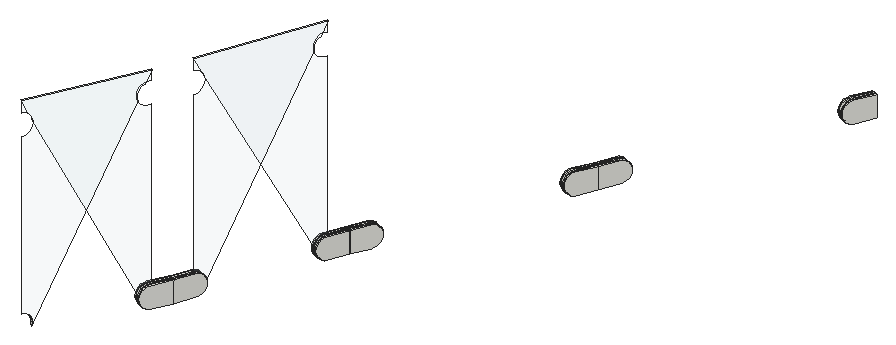
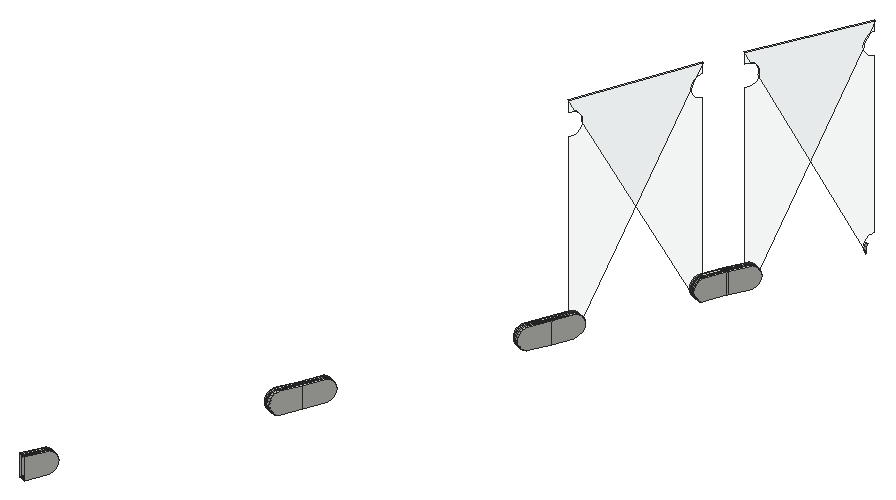
# SketchUp Ruby script. Lengths in inches.
U = 1.inch
M = Sketchup.active_model
def pt(a) = Geom::Point3d.new(a.map { |v| v * U })
def face(e, loops, mat)
  f = e.add_face(loops[0].map { |a| pt(a) })
  loops[1..].each { |l| e.add_face(l.map { |a| pt(a) }).erase! }
  f.material = f.back_material = mat if mat
  f
end
# faces: each face lists its corners as indices into pts; further lists are holes
def faces(e, pts, list, mat = nil) = list.each { |f| face(e, (f[0].is_a?(Array) ? f : [f]).map { |l| l.map { |i| pts[i] } }, mat) }
# xy, xz, yz: faces in a plane at the given z, y or x. An outline is a flat list of corners, or four numbers for a rectangle; further outlines are holes
def ring(l) = l.size == 4 ? [[l[0], l[1]], [l[2], l[1]], [l[2], l[3]], [l[0], l[3]]] : l.each_slice(2).to_a
def flat(e, list, mat, &to3) = list.each { |f| face(e, (f[0].is_a?(Array) ? f : [f]).map { |l| ring(l).map { |u, v| to3.(u, v) } }, mat) }
def xy(e, z, list, mat = nil) = flat(e, list, mat) { |x, y| [x, y, z] }
def xz(e, y, list, mat = nil) = flat(e, list, mat) { |x, z| [x, y, z] }
def yz(e, x, list, mat = nil) = flat(e, list, mat) { |y, z| [x, y, z] }
def lines(e, pts, list) = list.each { |a, b| e.add_line(pt(pts[a]), pt(pts[b])) }
# prism: a flat outline (further loops are holes) pulled along v
def prism(e, loops, v, mat = nil)
  f = face(e, loops, mat); d = Geom::Vector3d.new(v.map { |x| x * U })
  f.pushpull(f.normal.samedirection?(d) ? d.length : -d.length)
end
def box(e, o, s, mat = nil) = prism(e, [[o, [o[0] + s[0], o[1], o[2]], [o[0] + s[0], o[1] + s[1], o[2]], [o[0], o[1] + s[1], o[2]]]], [0, 0, s[2]], mat)
def at(x, y, z, deg = 0) = Geom::Transformation.translation(pt([x, y, z])) * Geom::Transformation.rotation(ORIGIN, Z_AXIS, deg.degrees)
def axes(o, x, y, z) = Geom::Transformation.new([*x, 0, *y, 0, *z, 0, *pt(o).to_a, 1])
def part(name) = M.definitions.add(name)
# library, detail: a bought-in or finely detailed component or shape, given as its bounding box
def library(name, o, s) = part(name).tap { |d| box(d.entities, o, s) }
def detail(e, o, s) = box(e.add_group.entities, o, s)
def put(e, d, t, mat = nil) = e.add_instance(d, t).tap { |i| i.material = mat if mat }
def group(e, t, mat = nil) = e.add_group.tap { |g| g.transformation = t; g.material = mat if mat }.entities
root = M.entities
M.materials.add("Glass_Safety_01").color = [204, 235, 244]
M.materials["Glass_Safety_01"].alpha = 0.1
xy(root,333,[[882.822,624.661,882.573,624.779,882.681,625.009,883.414,626.559,883.663,626.441],[882.395,624.863,882.145,624.981,882.977,626.738,883.233,626.637,882.503,625.093],[883.672,626.464,883.416,626.565,884.14,628.396,884.396,628.294],[883.233,626.637,882.977,626.738,882.981,626.75,882.986,626.761,883.236,626.643],[883.236,626.643,882.986,626.761,883.7,628.569,883.957,628.468],
  [888.84,639.54,888.584,639.641,888.672,639.866,889.306,641.468,889.558,641.358],[888.4,639.713,888.144,639.814,888.868,641.645,889.124,641.544,888.489,639.938],[889.558,641.358,889.306,641.468,889.307,641.472,889.563,641.37,889.561,641.364],[889.563,641.37,889.307,641.472,890.092,643.273,890.344,643.163],[889.125,641.547,888.873,641.657,889.659,643.462,889.911,643.352],
  [897.674,659.993,897.421,660.103,897.491,660.262,898.207,661.907,898.46,661.797],[897.241,660.181,896.988,660.291,897.774,662.096,898.027,661.986,897.31,660.341],[898.46,661.797,898.207,661.907,898.994,663.712,899.246,663.602],[898.027,661.986,897.774,662.096,898.56,663.901,898.813,663.791],[907.619,682.827,907.367,682.937,907.429,683.08,908.153,684.742,908.405,684.632],
  [907.186,683.016,906.933,683.126,907.719,684.93,907.972,684.82,907.248,683.158]])
xy(root,333.078,[[882.741,625.135,882.563,625.219,883.233,626.637,883.325,626.601,883.414,626.559],[883.416,626.565,883.325,626.601,883.236,626.643,883.812,628.102,883.995,628.029],[883.325,626.601,883.233,626.637,883.234,626.64,883.236,626.643],[888.728,640.007,888.545,640.079,889.124,641.544,889.215,641.508,889.306,641.468],[889.306,641.468,889.215,641.508,889.307,641.472,889.306,641.47],
  [889.307,641.472,889.215,641.508,889.125,641.547,889.754,642.991,889.935,642.912],[897.579,660.464,897.398,660.542,898.027,661.986,898.207,661.907],[898.207,661.907,898.027,661.986,898.656,663.43,898.836,663.351],[907.524,683.298,907.343,683.377,907.972,684.82,908.153,684.742]],"Glass_Safety_01")
xy(root,335.047,[[882.741,625.135,883.414,626.559,883.325,626.601,883.233,626.637,882.563,625.219],[883.416,626.565,883.995,628.029,883.812,628.102,883.236,626.643,883.325,626.601],[883.325,626.601,883.236,626.643,883.234,626.64,883.233,626.637],[888.728,640.007,889.306,641.468,889.215,641.508,889.124,641.544,888.545,640.079],[889.306,641.468,889.306,641.47,889.307,641.472,889.215,641.508],
  [889.307,641.472,889.935,642.912,889.754,642.991,889.125,641.547,889.215,641.508],[897.579,660.464,898.207,661.907,898.027,661.986,897.398,660.542],[898.207,661.907,898.836,663.351,898.656,663.43,898.027,661.986]],"Glass_Safety_01")
xy(root,335.126,[[882.822,624.661,883.663,626.441,883.414,626.559,882.681,625.009,882.573,624.779],[882.395,624.863,882.503,625.093,883.233,626.637,882.977,626.738,882.145,624.981],[883.672,626.464,884.396,628.294,884.14,628.396,883.416,626.565],[883.233,626.637,883.236,626.643,882.986,626.761,882.981,626.75,882.977,626.738],[883.236,626.643,883.957,628.468,883.7,628.569,882.986,626.761],
  [888.84,639.54,889.558,641.358,889.306,641.468,888.672,639.866,888.584,639.641],[888.4,639.713,888.489,639.938,889.124,641.544,888.868,641.645,888.144,639.814],[889.558,641.358,889.561,641.364,889.563,641.37,889.307,641.472,889.306,641.468],[889.563,641.37,890.344,643.163,890.092,643.273,889.307,641.472],[889.125,641.547,889.911,643.352,889.659,643.462,888.873,641.657],
  [897.674,659.993,898.46,661.797,898.207,661.907,897.491,660.262,897.421,660.103],[897.241,660.181,897.31,660.341,898.027,661.986,897.774,662.096,896.988,660.291],[898.46,661.797,899.246,663.602,898.994,663.712,898.207,661.907],[898.027,661.986,898.813,663.791,898.56,663.901,897.774,662.096],[907.619,682.827,908.405,684.632,908.153,684.742,907.429,683.08,907.367,682.937],
  [907.186,683.016,907.248,683.158,907.972,684.82,907.719,684.93,906.933,683.126]])
p = [[883.663,626.441,335.126],[882.822,624.661,335.126],[882.704,624.413,335.089],[882.595,624.181,334.983],[882.501,623.982,334.814],[882.428,623.829,334.594],
  [882.383,623.733,334.338],[882.367,623.7,334.0625],[882.383,623.733,333.787],[882.428,623.829,333.531],[882.501,623.982,333.311],[882.595,624.181,333.142],
  [882.704,624.413,333.036],[882.822,624.661,333],[883.663,626.441,333],[882.573,624.779,335.126],[882.681,625.009,335.126],[882.681,625.009,333],
  [882.573,624.779,333],[882.455,624.53,333.036],[882.345,624.299,333.142],[882.251,624.1,333.311],[882.179,623.947,333.531],[882.134,623.851,333.787],
  [882.118,623.818,334.0625],[882.134,623.851,334.338],[882.179,623.947,334.594],[882.251,624.1,334.814],[882.345,624.299,334.983],[882.455,624.53,335.089],
  [882.395,624.863,333],[882.503,625.093,333],[883.233,626.637,333],[883.233,626.637,333.078],[883.233,626.637,335.047],[883.233,626.637,335.126],
  [882.503,625.093,335.126],[882.395,624.863,335.126],[882.277,624.615,335.089],[882.167,624.383,334.983],[882.073,624.184,334.814],[882.001,624.031,334.594],
  [881.962,623.948,334.371],[881.956,623.935,334.338],[881.94,623.902,334.0625],[881.956,623.935,333.787],[882.001,624.031,333.531],[882.073,624.184,333.311],
  [882.167,624.383,333.142],[882.248,624.553,333.064],[882.277,624.615,333.036],[882.145,624.981,335.126],[882.977,626.738,335.126],[882.977,626.738,333],
  [882.145,624.981,333],[882.028,624.732,333.036],[881.918,624.501,333.142],[881.824,624.301,333.311],[881.752,624.149,333.531],[881.707,624.053,333.787],
  [881.691,624.02,334.0625],[881.707,624.053,334.338],[881.752,624.149,334.594],[881.824,624.301,334.814],[881.918,624.501,334.983],[882.028,624.732,335.089],
  [883.414,626.559,333],[883.414,626.559,335.126],[883.414,626.559,335.047],[882.741,625.135,335.047],[882.741,625.135,333.078],[883.414,626.559,333.078],
  [883.416,626.565,333.078],[883.416,626.565,333],[883.672,626.464,333],[883.672,626.464,335.126],[883.416,626.565,335.126],[883.416,626.565,335.047],
  [884.396,628.294,335.126],[884.396,628.294,333],[884.497,628.55,333.036],[884.591,628.789,333.142],[884.672,628.993,333.311],[884.734,629.15,333.531],
  [884.773,629.249,333.787],[884.787,629.283,334.0625],[884.773,629.249,334.338],[884.734,629.15,334.594],[884.672,628.993,334.814],[884.591,628.789,334.983],
  [884.497,628.55,335.089],[883.236,626.643,333.078],[883.236,626.643,333],[882.986,626.761,333],[882.986,626.761,335.126],[883.236,626.643,335.126],
  [883.236,626.643,335.047],[883.957,628.468,333],[884.058,628.724,333.036],[884.152,628.962,333.142],[884.233,629.167,333.311],[884.295,629.324,333.531],
  [884.334,629.423,333.787],[884.347,629.456,334.0625],[884.334,629.423,334.338],[884.295,629.324,334.594],[884.233,629.167,334.814],[884.152,628.962,334.983],
  [884.058,628.724,335.089],[883.957,628.468,335.126],[884.14,628.396,335.126],[884.14,628.396,333],[883.995,628.029,333.078],[883.995,628.029,335.047],
  [882.981,626.75,333],[882.981,626.75,335.126],[883.7,628.569,335.126],[883.801,628.825,335.089],[883.896,629.063,334.983],[883.977,629.268,334.814],
  [884.039,629.425,334.594],[884.078,629.524,334.338],[884.091,629.558,334.0625],[884.078,629.524,333.787],[884.039,629.425,333.531],[883.977,629.268,333.311],
  [883.896,629.063,333.142],[883.801,628.825,333.036],[883.7,628.569,333],[884.241,628.651,333.036],[884.512,629.338,333.756],[884.44,629.157,333.398],
  [884.416,629.095,333.311],[884.335,628.89,333.142],[884.241,628.651,335.089],[884.335,628.89,334.983],[884.416,629.095,334.814],[884.478,629.252,334.594],
  [884.517,629.35,334.338],[884.53,629.384,334.0625],[884.517,629.35,333.787],[888.84,639.54,333],[889.558,641.358,333],[889.558,641.358,335.126],
  [888.84,639.54,335.126],[888.739,639.284,335.089],[888.644,639.045,334.983],[888.564,638.84,334.814],[888.501,638.683,334.594],[888.462,638.585,334.338],
  [888.449,638.551,334.0625],[888.462,638.585,333.787],[888.501,638.683,333.531],[888.564,638.84,333.311],[888.644,639.045,333.142],[888.739,639.284,333.036],
  [888.489,639.938,333],[888.489,639.938,335.126],[888.4,639.713,335.126],[888.299,639.457,335.089],[888.205,639.219,334.983],[888.124,639.014,334.814],
  [888.062,638.857,334.594],[888.023,638.758,334.338],[888.019,638.747,334.245],[888.25,639.332,333.091],[888.299,639.457,333.036],[888.4,639.713,333],
  [888.672,639.866,333],[888.672,639.866,335.126],[888.584,639.641,335.126],[888.482,639.385,335.089],[888.388,639.147,334.983],[888.307,638.942,334.814],
  [888.245,638.785,334.594],[888.206,638.686,334.338],[888.193,638.652,334.0625],[888.206,638.686,333.787],[888.245,638.785,333.531],[888.307,638.942,333.311],
  [888.388,639.147,333.142],[888.482,639.385,333.036],[888.584,639.641,333],[889.306,641.468,335.126],[889.306,641.468,335.047],[889.306,641.468,333.078],
  [889.306,641.468,333],[888.144,639.814,335.126],[888.868,641.645,335.126],[888.868,641.645,333],[888.144,639.814,333],[888.043,639.559,333.036],
  [887.949,639.32,333.142],[887.868,639.115,333.311],[887.806,638.958,333.531],[887.767,638.86,333.787],[887.753,638.826,334.0625],[887.767,638.86,334.338],
  [887.806,638.958,334.594],[887.868,639.115,334.814],[887.949,639.32,334.983],[888.043,639.559,335.089],[888.205,639.219,333.142],[889.124,641.544,335.126],
  [889.124,641.544,333],[889.124,641.544,333.078],[888.545,640.079,333.078],[888.545,640.079,335.047],[889.124,641.544,335.047],[889.307,641.472,333],
  [889.307,641.472,333.078],[889.307,641.472,335.047],[889.307,641.472,335.126],[889.563,641.37,335.126],[889.563,641.37,333],[889.561,641.364,335.126],
  [889.561,641.364,333],[890.344,643.163,333],[890.454,643.415,333.036],[890.557,643.65,333.142],[890.645,643.852,333.311],[890.712,644.007,333.531],
  [890.754,644.105,333.787],[890.769,644.138,334.0625],[890.754,644.105,334.338],[890.712,644.007,334.594],[890.645,643.852,334.814],[890.557,643.65,334.983],
  [890.454,643.415,335.089],[890.344,643.163,335.126],[889.125,641.547,333],[889.125,641.547,333.078],[889.125,641.547,335.047],[889.125,641.547,335.126],
  [888.873,641.657,335.126],[888.873,641.657,333],[889.911,643.352,333],[889.911,643.352,335.126],[889.754,642.991,335.047],[889.754,642.991,333.078],
  [890.092,643.273,335.126],[890.202,643.525,335.089],[890.304,643.76,334.983],[890.392,643.962,334.814],[890.459,644.117,334.594],[890.502,644.215,334.338],
  [890.516,644.248,334.0625],[890.502,644.215,333.787],[890.459,644.117,333.531],[890.392,643.962,333.311],[890.304,643.76,333.142],[890.202,643.525,333.036],
  [890.092,643.273,333],[889.659,643.462,335.126],[889.768,643.714,335.089],[889.871,643.949,334.983],[889.959,644.151,334.814],[890.026,644.306,334.594],
  [890.069,644.403,334.338],[890.083,644.436,334.0625],[890.069,644.403,333.787],[890.026,644.306,333.531],[889.959,644.151,333.311],[889.871,643.949,333.142],
  [889.768,643.714,333.036],[889.659,643.462,333],[890.021,643.604,333.036],[890.021,643.604,335.089],[890.123,643.839,334.983],[890.211,644.041,334.814],
  [890.279,644.196,334.594],[890.321,644.293,334.338],[890.336,644.326,334.0625],[890.321,644.293,333.787],[890.279,644.196,333.531],[890.211,644.041,333.311],
  [890.123,643.839,333.142],[898.46,661.797,335.126],[897.674,659.993,335.126],[897.564,659.74,335.089],[897.462,659.505,334.983],[897.374,659.303,334.814],
  [897.307,659.149,334.594],[897.264,659.051,334.338],[897.25,659.018,334.0625],[897.264,659.051,333.787],[897.307,659.149,333.531],[897.374,659.303,333.311],
  [897.462,659.505,333.142],[897.564,659.74,333.036],[897.674,659.993,333],[898.46,661.797,333],[897.421,660.103,335.126],[897.491,660.262,335.126],
  [897.491,660.262,333],[897.421,660.103,333],[897.312,659.85,333.036],[897.209,659.615,333.142],[897.121,659.414,333.311],[897.054,659.259,333.531],
  [897.011,659.161,333.787],[896.997,659.128,334.0625],[897.011,659.161,334.338],[897.054,659.259,334.594],[897.121,659.414,334.814],[897.209,659.615,334.983],
  [897.312,659.85,335.089],[897.241,660.181,333],[897.31,660.341,333],[897.31,660.341,335.126],[897.241,660.181,335.126],[897.131,659.929,335.089],
  [897.029,659.694,334.983],[896.941,659.492,334.814],[896.873,659.337,334.594],[896.831,659.24,334.338],[896.817,659.207,334.0625],[896.831,659.24,333.787],
  [896.873,659.337,333.531],[896.941,659.492,333.311],[897.029,659.694,333.142],[897.131,659.929,333.036],[896.988,660.291,335.126],[897.774,662.096,335.126],
  [897.774,662.096,333],[896.988,660.291,333],[896.878,660.039,333.036],[896.776,659.804,333.142],[896.688,659.602,333.311],[896.621,659.447,333.531],
  [896.578,659.35,333.787],[896.564,659.317,334.0625],[896.578,659.35,334.338],[896.621,659.447,334.594],[896.688,659.602,334.814],[896.776,659.804,334.983],
  [896.878,660.039,335.089],[898.027,661.986,335.126],[898.027,661.986,333],[898.027,661.986,333.078],[897.398,660.542,333.078],[897.398,660.542,335.047],
  [898.027,661.986,335.047],[898.207,661.907,333],[898.207,661.907,335.126],[898.207,661.907,335.047],[897.579,660.464,335.047],[897.579,660.464,333.078],
  [898.207,661.907,333.078],[899.246,663.602,335.126],[899.246,663.602,333],[899.356,663.854,333.036],[899.458,664.089,333.142],[899.546,664.291,333.311],
  [899.614,664.446,333.531],[899.656,664.543,333.787],[899.671,664.577,334.0625],[899.656,664.543,334.338],[899.614,664.446,334.594],[899.546,664.291,334.814],
  [899.458,664.089,334.983],[899.356,663.854,335.089],[898.994,663.712,335.126],[898.994,663.712,333],[898.836,663.351,333.078],[898.836,663.351,335.047],
  [898.813,663.791,333],[898.813,663.791,335.126],[898.656,663.43,335.047],[898.656,663.43,333.078],[898.56,663.901,335.126],[898.67,664.153,335.089],
  [898.773,664.388,334.983],[898.86,664.59,334.814],[898.928,664.745,334.594],[898.97,664.842,334.338],[898.985,664.875,334.0625],[898.97,664.842,333.787],
  [898.928,664.745,333.531],[898.86,664.59,333.311],[898.773,664.388,333.142],[898.67,664.153,333.036],[898.56,663.901,333],[899.103,663.964,333.036],
  [899.206,664.199,333.142],[899.294,664.401,333.311],[899.361,664.556,333.531],[899.403,664.654,333.787],[899.418,664.687,334.0625],[899.403,664.654,334.338],
  [899.361,664.556,334.594],[899.294,664.401,334.814],[899.206,664.199,334.983],[899.103,663.964,335.089],[898.923,664.043,333.036],[898.923,664.043,335.089],
  [899.025,664.278,334.983],[899.113,664.48,334.814],[899.181,664.635,334.594],[899.223,664.732,334.338],[899.237,664.765,334.0625],[899.223,664.732,333.787],
  [899.181,664.635,333.531],[899.113,664.48,333.311],[899.025,664.278,333.142],[908.405,684.632,335.126],[907.619,682.827,335.126],[907.509,682.575,335.089],
  [907.407,682.34,334.983],[907.319,682.138,334.814],[907.252,681.983,334.594],[907.209,681.886,334.338],[907.195,681.852,334.0625],[907.209,681.886,333.787],
  [907.252,681.983,333.531],[907.319,682.138,333.311],[907.407,682.34,333.142],[907.509,682.575,333.036],[907.619,682.827,333],[908.405,684.632,333],
  [907.186,683.016,333],[907.248,683.158,333],[907.248,683.158,335.126],[907.186,683.016,335.126],[907.076,682.763,335.089],[906.974,682.528,334.983],
  [906.886,682.326,334.814],[906.818,682.172,334.594],[906.776,682.074,334.338],[906.762,682.041,334.0625],[906.776,682.074,333.787],[906.818,682.172,333.531],
  [906.886,682.326,333.311],[906.974,682.528,333.142],[907.076,682.763,333.036],[907.367,682.937,335.126],[907.429,683.08,335.126],[907.429,683.08,333],
  [907.367,682.937,333],[907.257,682.685,333.036],[907.154,682.45,333.142],[907.066,682.248,333.311],[906.999,682.093,333.531],[906.957,681.996,333.787],
  [906.942,681.962,334.0625],[906.957,681.996,334.338],[906.999,682.093,334.594],[907.066,682.248,334.814],[907.154,682.45,334.983],[907.257,682.685,335.089],
  [906.933,683.126,335.126],[907.719,684.93,335.126],[907.719,684.93,333],[906.933,683.126,333],[906.824,682.873,333.036],[906.721,682.638,333.142],
  [906.633,682.437,333.311],[906.566,682.282,333.531],[906.523,682.184,333.787],[906.509,682.151,334.0625],[906.523,682.184,334.338],[906.566,682.282,334.594],
  [906.633,682.437,334.814],[906.721,682.638,334.983],[906.824,682.873,335.089],[908.153,684.742,333],[908.153,684.742,335.126],[908.153,684.742,335.047],
  [907.524,683.298,335.047],[907.524,683.298,333.078],[908.153,684.742,333.078],[907.972,684.82,335.126],[907.972,684.82,333],[907.972,684.82,333.078],
  [907.343,683.377,333.078],[907.343,683.377,335.047],[907.972,684.82,335.047],[882.563,625.219,335.047],[882.563,625.219,333.078],[883.325,626.601,333.078],
  [883.325,626.601,335.047],[883.234,626.64,335.047],[883.234,626.64,333.078],[883.812,628.102,333.078],[883.812,628.102,335.047],[888.01,638.725,334.0625],
  [888.023,638.758,333.787],[888.062,638.857,333.531],[888.124,639.014,333.311],[888.728,640.007,333.078],[888.728,640.007,335.047],[889.215,641.508,335.047],
  [889.215,641.508,333.078],[889.306,641.47,333.078],[889.306,641.47,335.047],[889.935,642.912,335.047],[889.935,642.912,333.078],[884.478,629.252,333.531],
  [878.01,615.586,334.0625],[877.995,615.553,333.787],[877.745,615.671,333.787],[877.761,615.704,334.0625],[884.14,628.396,351.283],[888.202,638.675,352.163],
  [888.193,638.652,352.346],[888.206,638.686,352.621],[888.245,638.785,352.877],[888.307,638.942,353.098],[888.388,639.147,353.267],[888.433,639.26,353.317],
  [888.672,639.866,354.511],[884.14,628.396,354.511],[884.14,628.396,353.409],[884.241,628.651,353.373],[884.335,628.89,353.267],[884.416,629.095,353.098],
  [884.478,629.252,352.877],[884.517,629.35,352.621],[884.53,629.384,352.346],[884.517,629.35,352.071],[884.478,629.252,351.814],[884.416,629.095,351.594],
  [884.335,628.89,351.425],[884.241,628.651,351.319],[878.181,615.487,333.943],[882.14,623.863,352.037],[882.134,623.851,352.071],[882.118,623.818,352.346],
  [882.134,623.851,352.621],[882.179,623.947,352.877],[882.251,624.1,353.098],[882.345,624.299,353.267],[882.426,624.469,353.344],[882.681,625.009,354.511],
  [877.734,614.541,354.511],[877.734,614.541,353.409],[877.851,614.789,353.373],[877.961,615.021,353.267],[878.055,615.22,353.098],[878.127,615.373,352.877],
  [878.173,615.469,352.621],[878.188,615.502,352.346],[878.173,615.469,352.071],[878.127,615.373,351.814],[878.055,615.22,351.594],[877.961,615.021,351.425],
  [877.851,614.789,351.319],[877.734,614.541,351.283],[877.734,614.541,335.126],[877.851,614.789,335.089],[877.961,615.021,334.983],[878.055,615.22,334.814],
  [878.127,615.373,334.594],[878.173,615.469,334.338],[878.188,615.502,334.0625],[877.995,615.553,334.338],[877.745,615.671,334.338],[884.329,629.411,352.653],
  [884.295,629.324,352.877],[884.257,629.229,353.01],[883.957,628.468,354.511],[888.489,639.938,354.511],[888.489,639.938,353.409],[888.4,639.713,353.409],
  [888.299,639.457,353.373],[888.205,639.219,353.267],[888.124,639.014,353.098],[888.062,638.857,352.877],[888.023,638.758,352.621],[888.01,638.725,352.346],
  [888.023,638.758,352.071],[888.062,638.857,351.814],[888.124,639.014,351.594],[888.205,639.219,351.425],[888.299,639.457,351.319],[888.4,639.713,351.283],
  [888.489,639.938,351.283],[877.949,615.457,334.594],[877.7,615.575,334.594],[878.003,615.572,352.466],[877.995,615.553,352.621],[877.949,615.457,352.877],
  [877.877,615.304,353.098],[877.857,615.263,353.133],[877.556,614.625,354.511],[882.503,625.093,354.511],[882.503,625.093,353.409],[882.395,624.863,353.409],
  [882.277,624.615,353.373],[882.167,624.383,353.267],[882.073,624.184,353.098],[882.001,624.031,352.877],[881.956,623.935,352.621],[881.94,623.902,352.346],
  [881.956,623.935,352.071],[882.001,624.031,351.814],[882.073,624.184,351.594],[882.167,624.383,351.425],[882.277,624.615,351.319],[882.395,624.863,351.283],
  [882.503,625.093,351.283]]
faces(root,p,[[0,1,2,3,4,5,6,7,8,9,10,11,12,13,14],[15,16,17,18,19,20,21,22,23,24,25,26,27,28,29],[30,31,32,33,34,35,36,37,38,39,40,41,42,43,44,45,46,47,48,49,50],[51,52,53,54,55,56,57,58,59,60,61,62,63,64,65],[20,19,12,11],[49,48,56,55,50],[19,18,13,12],[30,50,55,54],
  [66,17,16,67,68,69,70,71],[66,71,68,67,0,14],[72,73,74,75,76,77],[78,75,74,79,80,81,82,83,84,85,86,87,88,89,90],[32,33,34,35,52,53],[91,92,93,94,95,96],[95,35,34,33,32,92,91,96],[95,35,34,33,32,92,97,98,99,100,101,102,103,104,105,106,107,108,109],
  [76,110,111,73,72,112,113,77],[114,53,52,115,94,93],[52,115,94,116,117,118,119,120,121,122,123,124,125,126,127,128,93,114,53],[111,129,80,79],[98,97,128,127],[129,133,81,80],[99,98,127,126],[141,142,143,144,145,146,147,148,149,150,151,152,153,154,155],
  [169,183,184,185,186,168,182,181,180,179,178,177,176,175,174,173,172,171,170],[187,188,189,190,191,192,193,194,195,196,197,198,199,200,201],[180,181,155,154],[165,202,192,191,166],[181,182,141,155],[167,166,191,190],[203,157,156,204,205,206,207,208],[185,186,142,143,183,184],
  [209,210,211,212,213,214],[215,143,142,216,214,213],[215,143,142,216,214,217,218,219,220,221,222,223,224,225,226,227,228,229,213],[205,204,189,188,203,208],[230,231,232,233,234,235],[230,236,237,233,232,238,239,231],[209,186,185,184,183,212,211,210],[183,212,240,241,242,243,244,245,246,247,248,249,250,251,252,209,186,185,184],
  [234,253,254,255,256,257,258,259,260,261,262,263,264,265,235],[252,251,218,217],[266,236,265,264],[251,250,219,218],[276,266,264,263],[277,278,279,280,281,282,283,284,285,286,287,288,289,290,291],[292,293,294,295,296,297,298,299,300,301,302,303,304,305,306],[307,308,309,310,311,312,313,314,315,316,317,318,319,320,321],
  [322,323,324,325,326,327,328,329,330,331,332,333,334,335,336],[297,296,289,288],[321,320,327,326],[296,295,290,289],[307,321,326,325],[337,309,308,338,339,340,341,342],[343,294,293,344,345,346,347,348],[343,348,345,344,277,291],
  [349,277,291,350,351,352,353,354,355,356,357,358,359,360,361],[344,362,363,343,348,364,365,345],[339,338,324,323,337,342],[338,366,367,337,342,368,369,339],[323,370,371,372,373,374,375,376,377,378,379,380,381,382,324],[363,383,351,350],[394,366,382,381],[383,384,352,351],
  [404,394,381,380],[405,406,407,408,409,410,411,412,413,414,415,416,417,418,419],[420,421,422,423,424,425,426,427,428,429,430,431,432,433,434],[435,436,437,438,439,440,441,442,443,444,445,446,447,448,449],[450,451,452,453,454,455,456,457,458,459,460,461,462,463,464],[440,439,417,416],[434,433,455,454],[439,438,418,417],
  [420,434,454,453],[465,437,436,466,467,468,469,470],[471,422,421,472,473,474,475,476],[21,20,11,10],[48,47,57,56],[133,132,82,81],[100,99,126,125],[164,485,486,487,488,202,165],
  [179,180,154,153],[202,488,193,192],[250,249,220,219],[275,276,263,262],[298,297,288,287],[320,319,328,327],[384,385,353,352],[403,404,380,379],
  [441,440,416,415],[433,432,456,455],[22,21,10,9],[47,46,58,57],[131,497,83,82,132],[101,100,125,124],[178,179,153,152],[488,487,194,193],
  [249,248,221,220],[274,275,262,261],[299,298,287,286],[319,318,329,328],[385,386,354,353],[402,403,379,378],[442,441,415,414],[432,431,457,456],
  [23,22,9,8],[46,45,59,58],[130,140,84,83,497],[102,101,124,123],[177,178,152,151],[487,486,195,194],[248,247,222,221],[273,274,261,260],
  [300,299,286,285],[318,317,330,329],[386,387,355,354],[401,402,378,377],[443,442,414,413],[431,430,458,457],[498,499,500,501],[24,23,8,7],
  [45,44,60,59],[140,139,85,84],[103,102,123,122],[176,177,151,150],[486,485,196,195],[247,246,223,222],[272,273,260,259],[301,300,285,284],
  [317,316,331,330],[387,388,356,355],[400,401,377,376],[444,443,413,412],[430,429,459,458],[555,498,501,556],[25,24,7,6],[44,43,61,60],
  [139,138,86,85],[104,103,122,121],[175,176,150,149],[164,163,197,196,485],[246,245,224,223],[271,272,259,258],[302,301,284,283],[316,315,332,331],
  [388,389,357,356],[399,400,376,375],[445,444,412,411],[429,428,460,459],[577,555,556,578],[26,25,6,5],[42,41,62,61,43],[138,137,87,86],
  [105,104,121,120],[174,175,149,148],[163,162,198,197],[245,244,225,224],[270,271,258,257],[303,302,283,282],[315,314,333,332],[389,390,358,357],
  [398,399,375,374],[446,445,411,410],[428,427,461,460],[27,26,5,4],[41,40,63,62],[137,136,88,87],[106,105,120,119],[173,174,148,147],
  [162,161,199,198],[244,243,226,225],[269,270,257,256],[304,303,282,281],[314,313,334,333],[390,391,359,358],[397,398,374,373],[447,446,410,409],
  [427,426,462,461],[28,27,4,3],[40,39,64,63],[136,135,89,88],[107,106,119,118],[172,173,147,146],[161,160,200,199],[243,242,227,226],
  [268,269,256,255],[305,304,281,280],[313,312,335,334],[391,392,360,359],[396,397,373,372],[448,447,409,408],[426,425,463,462],[29,28,3,2],
  [39,38,65,64],[135,134,90,89],[108,107,118,117],[171,172,146,145],[160,159,201,200],[242,241,228,227],[267,268,255,254],[306,305,280,279],
  [312,311,336,335],[392,393,361,360],[395,396,372,371],[449,448,408,407],[425,424,464,463],[15,29,2,1],[38,37,51,65],[134,110,78,90],
  [109,108,117,116],[170,171,145,144],[159,158,187,201],[241,240,229,228],[237,267,254,253],[292,306,279,278],[311,310,322,336],[393,362,349,361],
  [367,395,371,370],[435,449,407,406],[424,423,450,464]])
faces(root,p,[[130,131,132,133,129,111,110,134,135,136,137,138,139,140],[97,109,108,107,106,105,104,103,102,101,100,99,98],[156,157,158,159,160,161,162,163,164,165,166,167],[168,169,170,171,172,173,174,175,176,177,178,179,180,181,182],[240,252,251,250,249,248,247,246,245,244,243,242,241],[236,237,267,268,269,270,271,272,273,274,275,276,266],[362,363,383,384,385,386,387,388,389,390,391,392,393],[366,367,395,396,397,398,399,400,401,402,403,404,394],
  [42,49,48,47,46,45,44,43],[70,69,477,478],[71,70,69,68],[477,34,33,478],[479,480,34,33],[96,480,479,91],[481,96,91,482,33,34],[483,91,96,484],
  [71,479,480,68],[480,479,72,77],[112,72,77,113],[112,483,484,113],[489,490,207,206],[489,185,184,490],[206,205,208,207],[208,491,492,205],
  [492,491,232,231],[231,239,238,232],[491,492,185,184],[210,492,491,211],[493,210,211,494,184,185],[495,211,210,496],[238,495,496,239],[347,346,341,340],
  [340,339,342,341],[348,347,346,345],[342,345,348,339],[364,348,345,365],[339,369,368,342],[365,364,369,368],[469,468,475,474],[470,469,468,467],
  [130,131,497],[502,110,134,135,136,137,138,139,140,130,503,504,505,506,507,508,509,510,511,512,513,514,515,516,517,518,519,520,521,522,523],[524,525,526,527,528,529,530,531,532,533,534,535,536,537,538,539,540,541,542,543,544,545,546,547,548,549,550,551,552,553,554],[164,557,558,559,560,561,562,563,564,565,566,567,568,569,570,571,572,573,574,575,576,157,158,159,160,161,162,163],[42,579,580,581,582,583,584,585,586,587,588,589,590,591,592,593,594,595,596,597,598,599,600,36,37,38,39,40,41]],"Glass_Safety_01")
